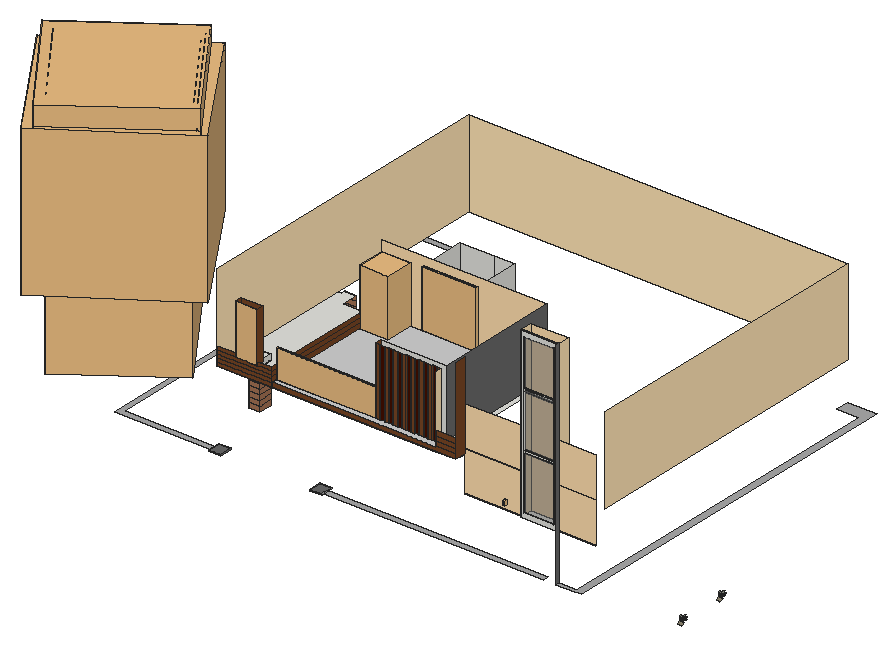
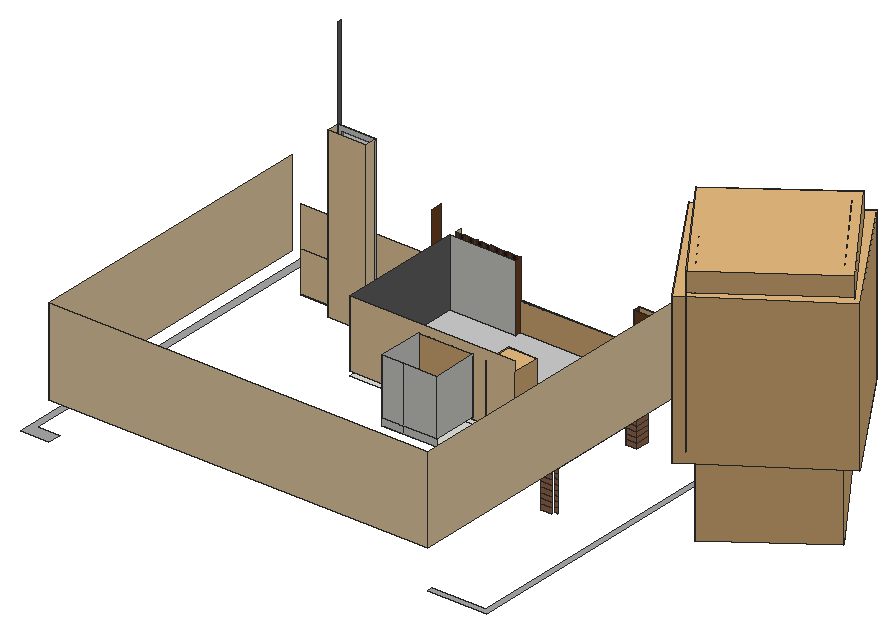
# SketchUp Ruby script. Lengths in inches.
U = 1.inch
M = Sketchup.active_model
def pt(a) = Geom::Point3d.new(a.map { |v| v * U })
def face(e, loops, mat)
  f = e.add_face(loops[0].map { |a| pt(a) })
  loops[1..].each { |l| e.add_face(l.map { |a| pt(a) }).erase! }
  f.material = f.back_material = mat if mat
  f
end
# faces: each face lists its corners as indices into pts; further lists are holes
def faces(e, pts, list, mat = nil) = list.each { |f| face(e, (f[0].is_a?(Array) ? f : [f]).map { |l| l.map { |i| pts[i] } }, mat) }
# xy, xz, yz: faces in a plane at the given z, y or x. An outline is a flat list of corners, or four numbers for a rectangle; further outlines are holes
def ring(l) = l.size == 4 ? [[l[0], l[1]], [l[2], l[1]], [l[2], l[3]], [l[0], l[3]]] : l.each_slice(2).to_a
def flat(e, list, mat, &to3) = list.each { |f| face(e, (f[0].is_a?(Array) ? f : [f]).map { |l| ring(l).map { |u, v| to3.(u, v) } }, mat) }
def xy(e, z, list, mat = nil) = flat(e, list, mat) { |x, y| [x, y, z] }
def xz(e, y, list, mat = nil) = flat(e, list, mat) { |x, z| [x, y, z] }
def yz(e, x, list, mat = nil) = flat(e, list, mat) { |y, z| [x, y, z] }
def lines(e, pts, list) = list.each { |a, b| e.add_line(pt(pts[a]), pt(pts[b])) }
# prism: a flat outline (further loops are holes) pulled along v
def prism(e, loops, v, mat = nil)
  f = face(e, loops, mat); d = Geom::Vector3d.new(v.map { |x| x * U })
  f.pushpull(f.normal.samedirection?(d) ? d.length : -d.length)
end
def box(e, o, s, mat = nil) = prism(e, [[o, [o[0] + s[0], o[1], o[2]], [o[0] + s[0], o[1] + s[1], o[2]], [o[0], o[1] + s[1], o[2]]]], [0, 0, s[2]], mat)
def at(x, y, z, deg = 0) = Geom::Transformation.translation(pt([x, y, z])) * Geom::Transformation.rotation(ORIGIN, Z_AXIS, deg.degrees)
def axes(o, x, y, z) = Geom::Transformation.new([*x, 0, *y, 0, *z, 0, *pt(o).to_a, 1])
def part(name) = M.definitions.add(name)
# library, detail: a bought-in or finely detailed component or shape, given as its bounding box
def library(name, o, s) = part(name).tap { |d| box(d.entities, o, s) }
def detail(e, o, s) = box(e.add_group.entities, o, s)
def put(e, d, t, mat = nil) = e.add_instance(d, t).tap { |i| i.material = mat if mat }
def group(e, t, mat = nil) = e.add_group.tap { |g| g.transformation = t; g.material = mat if mat }.entities
root = M.entities
M.materials.add("028_190k_fullGeometry_Material \#4").color = [120, 148, 64]
M.materials.add("Material \#1").color = [140, 140, 140]
M.materials.add("[0032_Moccasin]").color = [255, 228, 181]
M.materials.add("[0033_NavajoWhite]").color = [255, 222, 173]
M.materials.add("[0132_LightGray]").color = [169, 169, 169]
M.materials.add("[0134_DimGray]").color = [105, 105, 105]
M.materials.add("[0135_DarkGray]").color = [81, 81, 81]
M.materials.add("[Carrera Marble]").color = [207, 207, 207]
M.materials.add("[Color B08]").color = [68, 16, 0]
M.materials.add("[Tile Ceramic Multi]").color = [165, 115, 84]
M.materials.add("[Translucent Glass Gray]").color = [128, 128, 128]
M.materials["[Translucent Glass Gray]"].alpha = 0.5
M.materials.add("[Wood Veneer 01]").color = [120, 70, 37]
M.materials.add("viburnumbladsadfasdfad0w122").color = [125, 129, 119]
M.materials.add("viburnumbloem1asdfas0d1fas0d616w").color = [137, 130, 109]
c1 = part("Component\#315")
p = [[0.25,0,0],[2.05,0.01,0.35],[1.81,4.2,1.66],[0,4.19,1.3125]]
faces(c1.entities,p,[[0,1,2,3]],"viburnumbladsadfasdfad0w122")
c2 = part("viburnumblad2")
put(c2.entities,c1,axes([-19.23,-4.49,-32.18],[83.35428,0,0],[0,79.38502,0],[0,0,83.35428]))
c3 = part("Component\#333")
p = [[6.15,4.98,1.43],[0.18,5.1,1.71],[0,0.13,0.29],[5.97,0,0]]
faces(c3.entities,p,[[0,1,2,3]],"viburnumbloem1asdfas0d1fas0d616w")
c4 = library("028_190k_fullGeometry_0",[-319.99,-281.1,-2.15],[577.33,562.38,1159.36])
c5 = library("028_190k_fullGeometry_1",[-333.4,-281.7,421.48],[600.33,578.53,738.83])
c6 = library("028_190k_fullGeometry_2",[-3584003,-3264710,4041818.25],[6566285.5,6460741.75,7903602.75])
c7 = library("028_190k_fullGeometry_3",[-353.86,-324.57,405.22],[652.24,636.69,781.83])
c8 = part("028_190k_fullGeometry_4")
p = [[125.51,152.8,882.93],[125.36,152.82,883.01],[124.8,155.5625,881.05]]
faces(c8.entities,p,[[0,1,2]],"028_190k_fullGeometry_Material \#4")
c9 = part("028_190k_fullGeometry")
g1 = group(c9.entities,at(0,0,0))
put(g1,c4,axes([0,0,0],[0.18998,-0.26642,0],[0.26642,0.18998,0],[0,0,0.32722]))
put(g1,c5,axes([0,0,0],[0.18998,-0.26642,0],[0.26642,0.18998,0],[0,0,0.32722]))
put(g1,c6,axes([0,0,0],[0.00002,-0.00003,0],[0.00003,0.00002,0],[0,0,0.00003]))
put(g1,c7,axes([0,0,0],[0.18998,-0.26642,0],[0.26642,0.18998,0],[0,0,0.32722]))
put(g1,c8,axes([0,0,0],[0.18998,-0.26642,0],[0.26642,0.18998,0],[0,0,0.32722]))
c10 = part("Window")
xy(c10.entities,0,[[0,0,19.69,1.97]])
xy(c10.entities,1.97,[[1.97,0,17.72,0.79]])
xy(c10.entities,1.97,[[1.97,0.79,17.72,1.97]],"[Translucent Glass Gray]")
xy(c10.entities,24.8,[[1.97,0,17.72,0.79]])
xy(c10.entities,24.8,[[1.97,0.79,17.72,1.97]],"[Translucent Glass Gray]")
xy(c10.entities,25.98,[[1.97,0,17.72,0.79],[1.97,0.79,17.72,1.97]])
xy(c10.entities,48.03,[[1.97,0,17.72,1.97]])
xy(c10.entities,49.21,[[1.97,0,17.72,0.79]])
xy(c10.entities,49.21,[[1.97,0.79,17.72,1.97]],"[Translucent Glass Gray]")
xy(c10.entities,68.9,[[1.97,0,17.72,0.79]])
xy(c10.entities,68.9,[[1.97,0.79,17.72,1.97]],"[Translucent Glass Gray]")
xy(c10.entities,70.87,[[0,0,19.69,1.97]])
xz(c10.entities,0,[[[0,0,19.69,70.87],[1.97,1.97,17.72,68.9]]])
xz(c10.entities,0.79,[[1.97,1.97,17.72,24.8],[1.97,25.98,17.72,48.82],[1.97,49.21,17.72,68.9]],"[Translucent Glass Gray]")
xz(c10.entities,1.97,[[[0,0,19.69,70.87],[1.97,1.97,17.72,68.9]],[1.97,24.8,17.72,25.98],[1.97,48.03,17.72,49.21]])
yz(c10.entities,0,[[0,0,1.97,70.87]])
yz(c10.entities,1.97,[[0,1.97,0.79,24.8],[0,24.8,1.97,25.98],[0,25.98,0.79,48.03],[0.79,25.98,1.97,48.03],[0,48.03,1.97,49.21],
  [0,49.21,0.79,68.9]])
yz(c10.entities,1.97,[[0.79,1.97,1.97,24.8],[0.79,49.21,1.97,68.9]],"[Translucent Glass Gray]")
yz(c10.entities,17.72,[[0,1.97,0.79,24.8],[0,24.8,1.97,25.98],[0,25.98,0.79,48.03],[0.79,25.98,1.97,48.03],[0,48.03,1.97,49.21],
  [0,49.21,0.79,68.9]])
yz(c10.entities,17.72,[[0.79,1.97,1.97,24.8],[0.79,49.21,1.97,68.9]],"[Translucent Glass Gray]")
yz(c10.entities,19.69,[[0,0,1.97,70.87]])
c11 = library("Lamp Wall Outdoor 94-02",[-1.89,-4.65,-3.17],[3.78,4.65,6.35])
c12 = library("Glass Railings(black Handrails)",[-57.04,-132.55,0],[169.29,2.52,28.17])
c13 = library("plant",[-22.43,-22.29,0],[44.86,44.58,89.56])
c14 = library("Entrance door assembly",[0,0,0],[5.91,53.15,95.28])
c15 = library("jali pattern 2",[0,0,0],[57.36,2,116.36])
xy(root,60,[[1491.42,218.5,1510.11,221.5],[1651.31,218.5,1669.62,221.5],[1491.42,221.5,1494.42,223.9375],[1494.42,221.5,1507.11,235.125],[1507.11,221.5,1510.11,238.125],
  [1651.31,221.5,1654.31,238.125],[1654.31,221.5,1666.62,235.125],[1666.62,221.5,1669.62,223.9375],[1491.42,223.9375,1494.42,231.9375],[1666.62,223.9375,1669.62,231.9375],
  [1491.42,231.9375,1494.42,238.125],[1666.62,231.9375,1669.62,235.125],[1494.42,235.125,1507.11,238.125],[1654.31,235.125,1669.62,238.125]])
xy(root,60,[[1338.625,223.9375,1491.42,223.9375,1491.42,231.9375,1346.625,231.9375,1346.625,799.5,1431.3125,799.5,1431.3125,807.5,1338.625,807.5],[1669.62,223.9375,2017.03,231.9375],[2036.3125,223.9375,2065.6875,223.9375,2076.625,224.21,2076.625,807.5,2031.3125,807.5,2031.3125,786.1875,2065.5625,786.1875,2065.5625,228.9375,2036.3125,228.9375]],"[0132_LightGray]")
xy(root,61.5,[[1897.5625,327.3125,1957.25,348.375]])
xy(root,62,[[1491.42,218.5,1510.11,238.125],[1651.31,218.5,1669.62,238.125]],"[0134_DimGray]")
xy(root,82.58,[[1632.125,529.87,1632.04,529.89,1632.06,529.91],[1632.125,529.87,1632.06,529.91,1632.13,529.89],[1632.125,529.87,1632.13,529.89,1632.21,529.87],[1632.21,529.87,1632.13,529.89,1632.21,529.89],[1632.21,529.87,1632.21,529.89,1632.29,529.89],
  [1632.04,529.89,1631.98,529.93,1632,529.94],[1632.04,529.89,1632,529.94,1632.06,529.91],[1632.21,529.89,1632.28,529.91,1632.29,529.89],[1632.29,529.89,1632.28,529.91,1632.36,529.93],[1632.28,529.91,1632.34,529.94,1632.36,529.93],
  [1631.98,529.93,1631.93,529.98,1631.96,529.99],[1631.98,529.93,1631.96,529.99,1632,529.94],[1632.36,529.93,1632.34,529.94,1632.4,529.98],[1632.34,529.94,1632.38,529.99,1632.4,529.98],[1631.93,529.98,1631.92,530.04,1631.94,530.04],
  [1631.93,529.98,1631.94,530.04,1631.96,529.99],[1632.4,529.98,1632.38,529.99,1632.42,530.04],[1632.38,529.99,1632.39,530.04,1632.42,530.04],[1631.92,530.04,1631.93,530.1,1631.96,530.1],[1631.92,530.04,1631.96,530.1,1631.94,530.04],
  [1632.39,530.04,1632.38,530.1,1632.4,530.1],[1632.39,530.04,1632.4,530.1,1632.42,530.04],[1631.93,530.1,1631.98,530.15,1632,530.14],[1631.93,530.1,1632,530.14,1631.96,530.1],[1632.38,530.1,1632.34,530.14,1632.36,530.15],
  [1632.38,530.1,1632.36,530.15,1632.4,530.1],[1632,530.14,1631.98,530.15,1632.06,530.18],[1632.34,530.14,1632.28,530.18,1632.29,530.19],[1632.34,530.14,1632.29,530.19,1632.36,530.15],[1631.98,530.15,1632.04,530.19,1632.06,530.18],
  [1632.06,530.18,1632.04,530.19,1632.13,530.2],[1632.28,530.18,1632.21,530.2,1632.21,530.21],[1632.28,530.18,1632.21,530.21,1632.29,530.19],[1632.04,530.19,1632.125,530.21,1632.13,530.2],[1632.13,530.2,1632.125,530.21,1632.21,530.2],
  [1632.21,530.2,1632.125,530.21,1632.21,530.21]],"Material \#1")
xy(root,82.59,[[1632.125,529.87,1632.13,529.89,1632.04,529.89],[1632.125,529.87,1632.21,529.87,1632.21,529.89],[1632.125,529.87,1632.21,529.89,1632.13,529.89],[1632.21,529.87,1632.28,529.91,1632.21,529.89],[1632.21,529.87,1632.29,529.89,1632.28,529.91],
  [1632.04,529.89,1632.06,529.91,1631.98,529.93],[1632.04,529.89,1632.13,529.89,1632.06,529.91],[1632.29,529.89,1632.34,529.94,1632.28,529.91],[1632.29,529.89,1632.36,529.93,1632.34,529.94],[1632.06,529.91,1632,529.94,1631.98,529.93],
  [1631.98,529.93,1632,529.94,1631.93,529.98],[1632.36,529.93,1632.38,529.99,1632.34,529.94],[1632.36,529.93,1632.4,529.98,1632.38,529.99],[1632,529.94,1631.96,529.99,1631.93,529.98],[1631.93,529.98,1631.96,529.99,1631.92,530.04],
  [1632.4,529.98,1632.39,530.04,1632.38,529.99],[1632.4,529.98,1632.42,530.04,1632.39,530.04],[1631.96,529.99,1631.94,530.04,1631.92,530.04],[1631.92,530.04,1631.94,530.04,1631.93,530.1],[1631.94,530.04,1631.96,530.1,1631.93,530.1],
  [1632.39,530.04,1632.42,530.04,1632.38,530.1],[1632.42,530.04,1632.4,530.1,1632.38,530.1],[1631.93,530.1,1631.96,530.1,1631.98,530.15],[1631.96,530.1,1632,530.14,1631.98,530.15],[1632.38,530.1,1632.4,530.1,1632.34,530.14],
  [1632.4,530.1,1632.36,530.15,1632.34,530.14],[1632,530.14,1632.04,530.19,1631.98,530.15],[1632,530.14,1632.06,530.18,1632.04,530.19],[1632.34,530.14,1632.36,530.15,1632.28,530.18],[1632.36,530.15,1632.29,530.19,1632.28,530.18],
  [1632.06,530.18,1632.125,530.21,1632.04,530.19],[1632.06,530.18,1632.13,530.2,1632.125,530.21],[1632.28,530.18,1632.29,530.19,1632.21,530.2],[1632.29,530.19,1632.21,530.21,1632.21,530.2],[1632.13,530.2,1632.21,530.21,1632.125,530.21],
  [1632.13,530.2,1632.21,530.2,1632.21,530.21]],"Material \#1")
xy(root,86.59,[[1632.125,529.87,1632.04,529.89,1632.13,529.89],[1632.125,529.87,1632.13,529.89,1632.21,529.89],[1632.125,529.87,1632.21,529.89,1632.21,529.87],[1632.21,529.87,1632.21,529.89,1632.28,529.91],[1632.21,529.87,1632.28,529.91,1632.29,529.89],
  [1632.04,529.89,1631.98,529.93,1632.06,529.91],[1632.04,529.89,1632.06,529.91,1632.13,529.89],[1632.29,529.89,1632.28,529.91,1632.34,529.94],[1632.29,529.89,1632.34,529.94,1632.36,529.93],[1632.06,529.91,1631.98,529.93,1632,529.94],
  [1631.98,529.93,1631.93,529.98,1632,529.94],[1632.36,529.93,1632.34,529.94,1632.38,529.99],[1632.36,529.93,1632.38,529.99,1632.4,529.98],[1632,529.94,1631.93,529.98,1631.96,529.99],[1631.93,529.98,1631.92,530.04,1631.96,529.99],
  [1632.4,529.98,1632.38,529.99,1632.39,530.04],[1632.4,529.98,1632.39,530.04,1632.42,530.04],[1631.96,529.99,1631.92,530.04,1631.94,530.04],[1631.92,530.04,1631.93,530.1,1631.94,530.04],[1631.94,530.04,1631.93,530.1,1631.96,530.1],
  [1632.39,530.04,1632.38,530.1,1632.42,530.04],[1632.42,530.04,1632.38,530.1,1632.4,530.1],[1631.93,530.1,1631.98,530.15,1631.96,530.1],[1631.96,530.1,1631.98,530.15,1632,530.14],[1632.38,530.1,1632.34,530.14,1632.4,530.1],
  [1632.4,530.1,1632.34,530.14,1632.36,530.15],[1632,530.14,1631.98,530.15,1632.04,530.19],[1632,530.14,1632.04,530.19,1632.06,530.18],[1632.34,530.14,1632.28,530.18,1632.36,530.15],[1632.36,530.15,1632.28,530.18,1632.29,530.19],
  [1632.06,530.18,1632.04,530.19,1632.125,530.21],[1632.06,530.18,1632.125,530.21,1632.13,530.2],[1632.28,530.18,1632.21,530.2,1632.29,530.19],[1632.29,530.19,1632.21,530.2,1632.21,530.21],[1632.13,530.2,1632.125,530.21,1632.21,530.21],
  [1632.13,530.2,1632.21,530.21,1632.21,530.2]],"Material \#1")
xy(root,86.6,[[1632.125,529.87,1632.06,529.91,1632.04,529.89],[1632.125,529.87,1632.13,529.89,1632.06,529.91],[1632.125,529.87,1632.21,529.87,1632.13,529.89],[1632.21,529.87,1632.21,529.89,1632.13,529.89],[1632.21,529.87,1632.29,529.89,1632.21,529.89],
  [1632.04,529.89,1632,529.94,1631.98,529.93],[1632.04,529.89,1632.06,529.91,1632,529.94],[1632.21,529.89,1632.29,529.89,1632.28,529.91],[1632.29,529.89,1632.36,529.93,1632.28,529.91],[1632.28,529.91,1632.36,529.93,1632.34,529.94],
  [1631.98,529.93,1631.96,529.99,1631.93,529.98],[1631.98,529.93,1632,529.94,1631.96,529.99],[1632.36,529.93,1632.4,529.98,1632.34,529.94],[1632.34,529.94,1632.4,529.98,1632.38,529.99],[1631.93,529.98,1631.94,530.04,1631.92,530.04],
  [1631.93,529.98,1631.96,529.99,1631.94,530.04],[1632.4,529.98,1632.42,530.04,1632.38,529.99],[1632.38,529.99,1632.42,530.04,1632.39,530.04],[1631.92,530.04,1631.94,530.04,1631.96,530.1],[1631.92,530.04,1631.96,530.1,1631.93,530.1],
  [1632.39,530.04,1632.4,530.1,1632.38,530.1],[1632.39,530.04,1632.42,530.04,1632.4,530.1],[1631.93,530.1,1631.96,530.1,1632,530.14],[1631.93,530.1,1632,530.14,1631.98,530.15],[1632.38,530.1,1632.36,530.15,1632.34,530.14],
  [1632.38,530.1,1632.4,530.1,1632.36,530.15],[1632,530.14,1632.06,530.18,1631.98,530.15],[1632.34,530.14,1632.29,530.19,1632.28,530.18],[1632.34,530.14,1632.36,530.15,1632.29,530.19],[1631.98,530.15,1632.06,530.18,1632.04,530.19],
  [1632.06,530.18,1632.13,530.2,1632.04,530.19],[1632.28,530.18,1632.21,530.21,1632.21,530.2],[1632.28,530.18,1632.29,530.19,1632.21,530.21],[1632.04,530.19,1632.13,530.2,1632.125,530.21],[1632.13,530.2,1632.21,530.2,1632.125,530.21],
  [1632.21,530.2,1632.21,530.21,1632.125,530.21]],"Material \#1")
xy(root,95.25,[[1583.17,528.0625,1636.42,560.625],[1668.92,528.0625,1708.73,550.875]])
xy(root,120,[[[1431.3125,309.8125,1431.3125,549.6875,1437.22,549.6875,1437.22,555,1454.9375,555,1454.9375,528.0625,1777.8125,528.0625,1777.8125,309.8125],[1457.08,340.22,1474.64,362.07]],[1777.8125,309.8125,1809.4375,322.5],[1457.08,340.22,1474.64,362.07],[1583.17,528.0625,1668.92,600.9375]])
xy(root,127,[[1518,309.8125,1777.8125,309.8125,1777.8125,319.48,1770.93,319.48,1770.93,319.875,1764.05,319.875,1764.05,319.48,1757.18,319.48,1757.18,319.875,1750.3,319.875,1750.3,319.48,1743.42,319.48,1743.42,319.875,1736.54,319.875,1736.54,319.48,1729.66,319.48,1729.66,319.875,1722.78,319.875,1722.78,319.48,1715.9,319.48,1715.9,319.875,1709.02,319.875,1709.02,319.48,1702.14,319.48,1702.14,319.875,1695.26,319.875,1695.26,319.48,1688.38,319.48,1688.38,319.875,1681.5,319.875,1681.5,319.48,1674.625,319.48,1674.625,330.25,1777.8125,330.25,1777.8125,528.0625,1518,528.0625]],"[Carrera Marble]")
xy(root,128.75,[[1457.08,340.22,1474.64,362.07]])
xy(root,130.8125,[[1583.17,528.0625,1636.42,600.9375],[1636.42,528.0625,1668.92,600.9375]])
xy(root,142.6,[[1460.375,309.8125,1494.3,320.75]],"[Wood Veneer 01]")
xz(root,218.5,[[1491.42,60,1510.11,62],[1651.31,60,1669.62,62]],"[0134_DimGray]")
xz(root,238.125,[[1491.42,60,1510.11,62]])
xz(root,238.125,[[1651.31,60,1669.62,62]],"[0134_DimGray]")
xz(root,309.8125,[[1431.3125,120,1518,125.65],[1518,120,1809.4375,120,1809.4375,127.53,1777.8125,127.53,1777.8125,127,1518,127],[1431.3125,125.65,1518,131.3],[1777.8125,127.53,1809.4375,135.07],[1431.3125,131.3,1518,136.95],
  [1777.8125,135.07,1809.4375,142.6],[1431.3125,136.95,1518,142.6],[1431.3125,142.6,1460.375,148.25],[1494.3,142.6,1518,148.25],[1777.8125,142.6,1809.4375,150.13]],"[Wood Veneer 01]")
xz(root,319.48,[[1674.625,127,1681.5,233],[1688.38,127,1695.26,233],[1702.14,127,1709.02,233],[1715.9,127,1722.78,233],[1729.66,127,1736.54,233],
  [1743.42,127,1750.3,233],[1757.18,127,1764.05,233],[1770.93,127,1777.8125,233]],"[Wood Veneer 01]")
xz(root,319.875,[[1681.5,127,1688.38,233],[1695.26,127,1702.14,233],[1709.02,127,1715.9,233],[1722.78,127,1729.66,233],[1736.54,127,1743.42,233],
  [1750.3,127,1757.18,233],[1764.05,127,1770.93,233]],"[Color B08]")
xz(root,320.75,[[1460.375,142.6,1494.3,221.7]],"[Wood Veneer 01]")
xz(root,327.3125,[[1809.4375,64.23,1897.5625,127.47],[1957.25,64.23,2017.03,127.47],[1809.4375,128.47,1897.5625,191.7],[1957.25,128.47,2017.03,191.7]],"[0033_NavajoWhite]")
xz(root,327.3125,[[1809.4375,63.23,1897.5625,64.23],[1957.25,63.23,2017.03,64.23],[1809.4375,127.47,1897.5625,128.47],[1957.25,127.47,2017.03,128.47]],"[0135_DarkGray]")
xz(root,330.25,[[1674.625,127,1777.8125,233]])
xz(root,340.22,[[1457.08,120,1474.64,128.75]])
xz(root,340.22,[[1457.08,56,1474.64,64],[1457.08,64,1474.64,72],[1457.08,72,1474.64,80],[1457.08,80,1474.64,88],[1457.08,88,1474.64,96],
  [1457.08,96,1474.64,104],[1457.08,104,1474.64,112],[1457.08,112,1474.64,120]],"[Tile Ceramic Multi]")
xz(root,348.375,[[1897.5625,61.5,1957.25,326.75]],"[0033_NavajoWhite]")
xz(root,362.07,[[1457.08,120,1474.64,128.75]])
xz(root,362.07,[[1457.08,56,1474.64,64],[1457.08,64,1474.64,72],[1457.08,72,1474.64,80],[1457.08,80,1474.64,88],[1457.08,88,1474.64,96],
  [1457.08,96,1474.64,104],[1457.08,104,1474.64,112],[1457.08,112,1474.64,120]],"[Tile Ceramic Multi]")
xz(root,528.0625,[[[1518,127,1777.8125,233],[1583.17,130.8125,1668.92,219.625]]],"[0033_NavajoWhite]")
xz(root,549.6875,[[1431.3125,56,1437.22,64],[1431.3125,64,1437.22,72],[1431.3125,72,1437.22,80],[1431.3125,80,1437.22,88],[1431.3125,88,1437.22,96],
  [1431.3125,96,1437.22,104],[1431.3125,104,1437.22,112],[1431.3125,112,1437.22,120]],"[Tile Ceramic Multi]")
xz(root,555,[[1437.22,56,1454.9375,64],[1437.22,64,1454.9375,72],[1437.22,72,1454.9375,80],[1437.22,80,1454.9375,88],[1437.22,88,1454.9375,96],
  [1437.22,96,1454.9375,104],[1437.22,104,1454.9375,112],[1437.22,112,1454.9375,120]],"[Tile Ceramic Multi]")
xz(root,600.9375,[[1583.17,120,1636.42,130.8125],[1636.42,120,1668.92,130.8125],[1583.17,130.8125,1636.42,219.625],[1636.42,130.8125,1668.92,219.625]])
xz(root,807.5,[[1431.3125,120,2031.3125,257]],"[0032_Moccasin]")
yz(root,1431.3125,[[309.8125,120,807.5,257]],"[0032_Moccasin]")
yz(root,1457.08,[[340.22,120,362.07,128.75]])
yz(root,1457.08,[[340.22,56,362.07,64],[340.22,64,362.07,72],[340.22,72,362.07,80],[340.22,80,362.07,88],[340.22,88,362.07,96],
  [340.22,96,362.07,104],[340.22,104,362.07,112],[340.22,112,362.07,120]],"[Tile Ceramic Multi]")
yz(root,1460.375,[[309.8125,142.6,320.75,221.7]],"[Wood Veneer 01]")
yz(root,1474.64,[[340.22,120,362.07,128.75]])
yz(root,1474.64,[[340.22,56,362.07,64],[340.22,64,362.07,72],[340.22,72,362.07,80],[340.22,80,362.07,88],[340.22,88,362.07,96],
  [340.22,96,362.07,104],[340.22,104,362.07,112],[340.22,112,362.07,120]],"[Tile Ceramic Multi]")
yz(root,1491.42,[[218.5,60,223.9375,62],[223.9375,60,231.9375,62],[231.9375,60,238.125,62]],"[0134_DimGray]")
yz(root,1494.3,[[309.8125,142.6,320.75,221.7]],"[Wood Veneer 01]")
yz(root,1510.11,[[218.5,60,238.125,62]],"[0134_DimGray]")
yz(root,1518,[[309.8125,120,309.8125,127,315.75,127]])
yz(root,1518,[[309.8125,127,528.0625,134.07],[309.8125,134.07,528.0625,141.13],[309.8125,141.13,528.0625,148.2]],"[Wood Veneer 01]")
yz(root,1583.17,[[528.0625,130.8125,600.9375,219.625]])
yz(root,1651.31,[[218.5,60,238.125,62]],"[0134_DimGray]")
yz(root,1668.92,[[528.0625,130.8125,600.9375,219.625]])
yz(root,1669.62,[[218.5,60,223.9375,62],[223.9375,60,231.9375,62],[231.9375,60,238.125,62]],"[0132_LightGray]")
yz(root,1674.625,[[319.48,127,330.25,233]],"[Wood Veneer 01]")
yz(root,1681.5,[[319.48,127,319.875,233]],"[Wood Veneer 01]")
yz(root,1688.38,[[319.48,127,319.875,233]],"[Wood Veneer 01]")
yz(root,1695.26,[[319.48,127,319.875,233]],"[Wood Veneer 01]")
yz(root,1702.14,[[319.48,127,319.875,233]],"[Wood Veneer 01]")
yz(root,1709.02,[[319.48,127,319.875,233]],"[Wood Veneer 01]")
yz(root,1715.9,[[319.48,127,319.875,233]],"[Wood Veneer 01]")
yz(root,1722.78,[[319.48,127,319.875,233]],"[Wood Veneer 01]")
yz(root,1729.66,[[319.48,127,319.875,233]],"[Wood Veneer 01]")
yz(root,1736.54,[[319.48,127,319.875,233]],"[Wood Veneer 01]")
yz(root,1743.42,[[319.48,127,319.875,233]],"[Wood Veneer 01]")
yz(root,1750.3,[[319.48,127,319.875,233]],"[Wood Veneer 01]")
yz(root,1757.18,[[319.48,127,319.875,233]],"[Wood Veneer 01]")
yz(root,1764.05,[[319.48,127,319.875,233]],"[Wood Veneer 01]")
yz(root,1770.93,[[319.48,127,319.875,233]],"[Wood Veneer 01]")
yz(root,1777.8125,[[309.8125,127,319.48,233]],"[0032_Moccasin]")
yz(root,1777.8125,[[330.25,127,528.0625,233]],"[0134_DimGray]")
yz(root,1809.4375,[[309.8125,120,327.3125,257]],"[Wood Veneer 01]")
yz(root,1897.5625,[[327.3125,61.5,348.375,326.75]],"[0032_Moccasin]")
yz(root,1957.25,[[327.3125,61.5,348.375,326.75]],"[0032_Moccasin]")
yz(root,2031.3125,[[327.5,120,807.5,257]],"[0032_Moccasin]")
yz(root,2036.3125,[[223.9375,60,228.9375,400.3125]],"[0134_DimGray]")
put(root,c2,axes([2205.85,342.29,51.46],[0,-0.01388,-0.00141],[0.01194,-0.00015,0.00146],[-0.00163,-0.00134,0.0132]))
put(root,c2,axes([2205.85,265.41,51.46],[0,-0.01388,-0.00141],[0.01194,-0.00015,0.00146],[-0.00163,-0.00134,0.0132]))
put(root,c2,axes([2206.74,341.16,51.44],[-0.01222,-0.00003,-0.00133],[0,-0.01336,0.00028],[-0.00144,0.00028,0.01328]))
put(root,c2,axes([2206.74,264.27,51.44],[-0.01222,-0.00003,-0.00133],[0,-0.01336,0.00028],[-0.00144,0.00028,0.01328]))
put(root,c2,axes([2204.55,341.21,51.3],[0.01283,0,0],[0,0.01408,0.0032],[0,-0.00296,0.01303]))
put(root,c2,axes([2204.55,264.33,51.3],[0.01283,0,0],[0,0.01408,0.0032],[0,-0.00296,0.01303]))
put(root,c2,axes([2206.32,340.11,52.84],[-0.00945,0.0094,0.00096],[-0.00947,-0.00959,0.00068],[0.00115,-0.00019,0.01331]))
put(root,c2,axes([2206.32,263.23,52.84],[-0.00945,0.0094,0.00096],[-0.00947,-0.00959,0.00068],[0.00115,-0.00019,0.01331]))
put(root,c2,axes([2206.32,341.99,53],[-0.00945,-0.0094,-0.00096],[0.00861,-0.00872,0.00062],[-0.00115,-0.00019,0.01331]))
put(root,c2,axes([2206.32,265.11,53],[-0.00945,-0.0094,-0.00096],[0.00861,-0.00872,0.00062],[-0.00115,-0.00019,0.01331]))
put(root,c2,axes([2204.75,341.87,53],[0.00945,-0.0094,-0.00096],[0.00985,0.00963,0.0027],[-0.00115,-0.00249,0.01308]))
put(root,c2,axes([2204.75,264.98,53],[0.00945,-0.0094,-0.00096],[0.00985,0.00963,0.0027],[-0.00115,-0.00249,0.01308]))
put(root,c2,axes([2204.625,340.36,52.875],[0.00945,0.0094,0.00096],[-0.00938,0.00917,0.00257],[0.00115,-0.00249,0.01308]))
put(root,c2,axes([2204.625,263.48,52.875],[0.00945,0.0094,0.00096],[-0.00938,0.00917,0.00257],[0.00115,-0.00249,0.01308]))
put(root,c3,axes([2207.61,327.19,52.5],[1.0472,0,0],[0,1.0472,0],[0,0,1.0472]))
put(root,c3,axes([2207.61,250.3125,52.5],[1.0472,0,0],[0,1.0472,0],[0,0,1.0472]))
put(root,c2,axes([2205.24,339.8,54.52],[0,0.0133,0.00135],[-0.01327,-0.00016,0.00162],[0.00163,-0.00134,0.0132]))
put(root,c2,axes([2205.24,262.91,54.52],[0,0.0133,0.00135],[-0.01327,-0.00016,0.00162],[0.00163,-0.00134,0.0132]))
put(root,c2,axes([2205.65,342.14,54.76],[0,-0.0133,-0.00135],[0.01327,-0.00016,0.00162],[-0.00163,-0.00134,0.0132]))
put(root,c2,axes([2205.65,265.25,54.76],[0,-0.0133,-0.00135],[0.01327,-0.00016,0.00162],[-0.00163,-0.00134,0.0132]))
put(root,c2,axes([2206.625,340.76,54.62],[-0.01337,0,0],[0,-0.01336,0.00028],[0,0.00028,0.01336]))
put(root,c2,axes([2206.625,263.88,54.62],[-0.01337,0,0],[0,-0.01336,0.00028],[0,0.00028,0.01336]))
put(root,c2,axes([2204.27,341.17,54.66],[0.01337,0,0],[0,0.01303,0.00296],[0,-0.00296,0.01303]))
put(root,c2,axes([2204.27,264.29,54.66],[0.01337,0,0],[0,0.01303,0.00296],[0,-0.00296,0.01303]))
put(root,c9,at(1237.28,365.45,60.7))
put(root,c10,axes([1897.5625,327.3125,61.5],[3,0,0],[0,1,0],[0,0,3.74297]))
put(root,c11,at(1568.42,528.0625,67.91))
put(root,c11,at(1874.39,327.3125,74.95))
put(root,c12,axes([1571.16,394.82,127],[0.92175,0,0],[0,0.57,0],[0,0,1.596]))
put(root,c13,at(1540.43,505.77,127))
put(root,c14,axes([1583.17,524.28,219.625],[0,0.64,0],[1.61337,0,0],[0,0,-0.94528]))
put(root,c15,axes([1460.375,309.8125,142.6],[0.59137,0,0],[0,0.36,0],[0,0,0.67979]))
